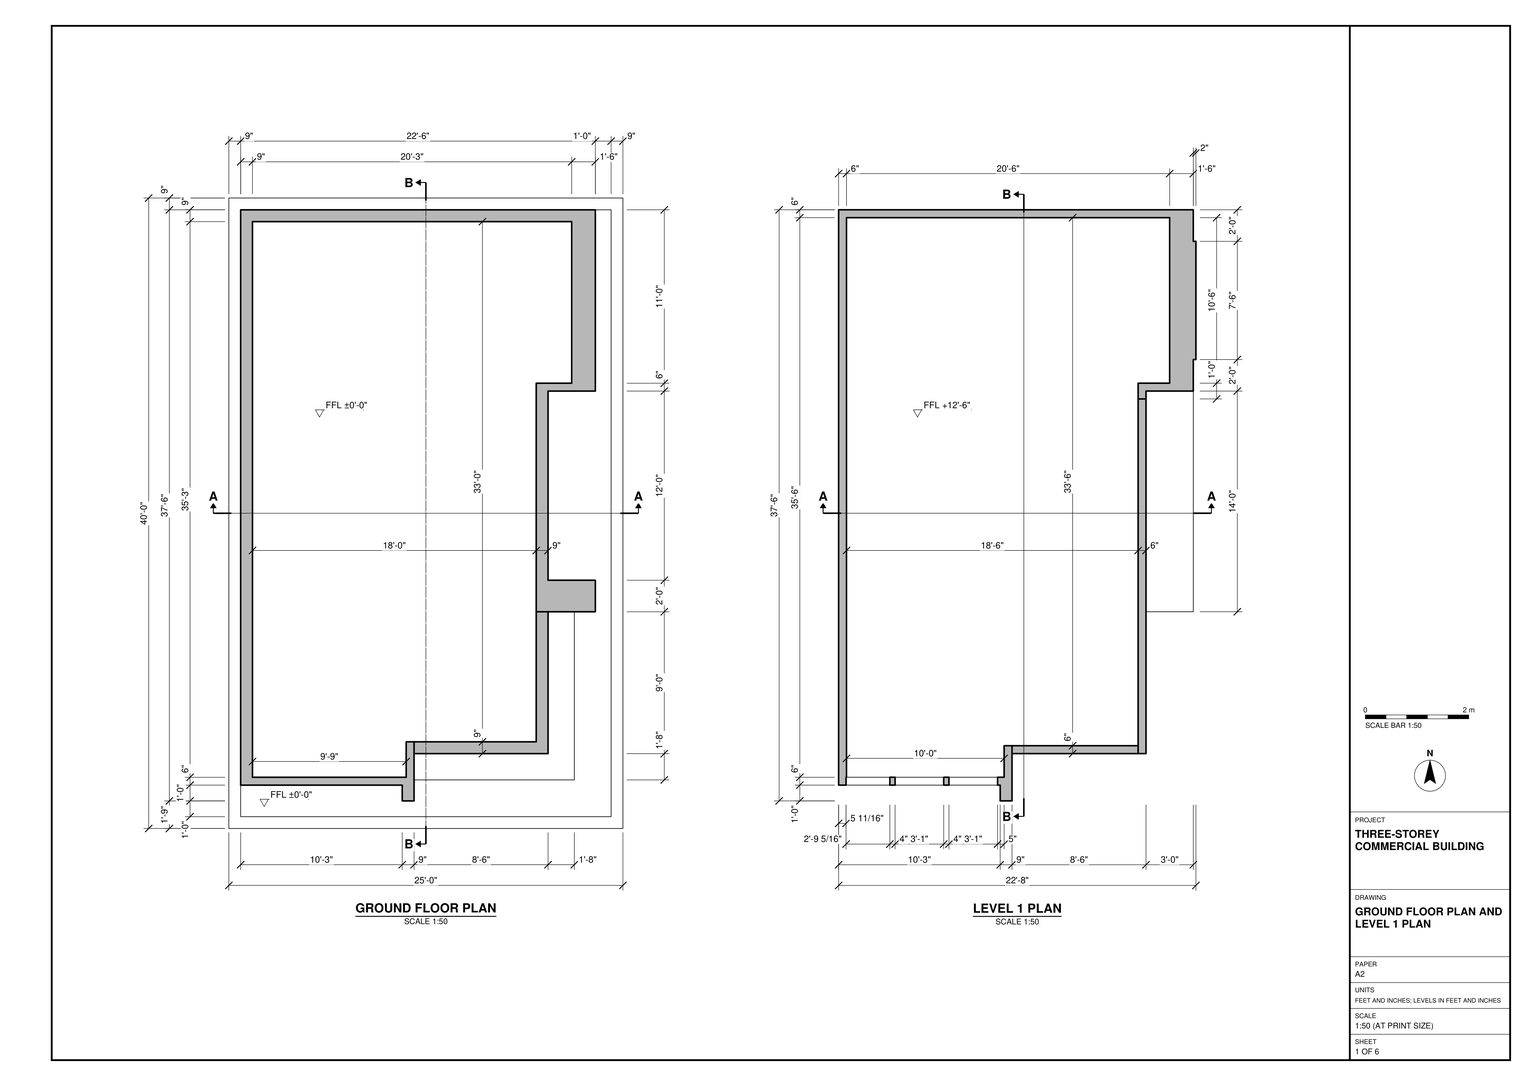
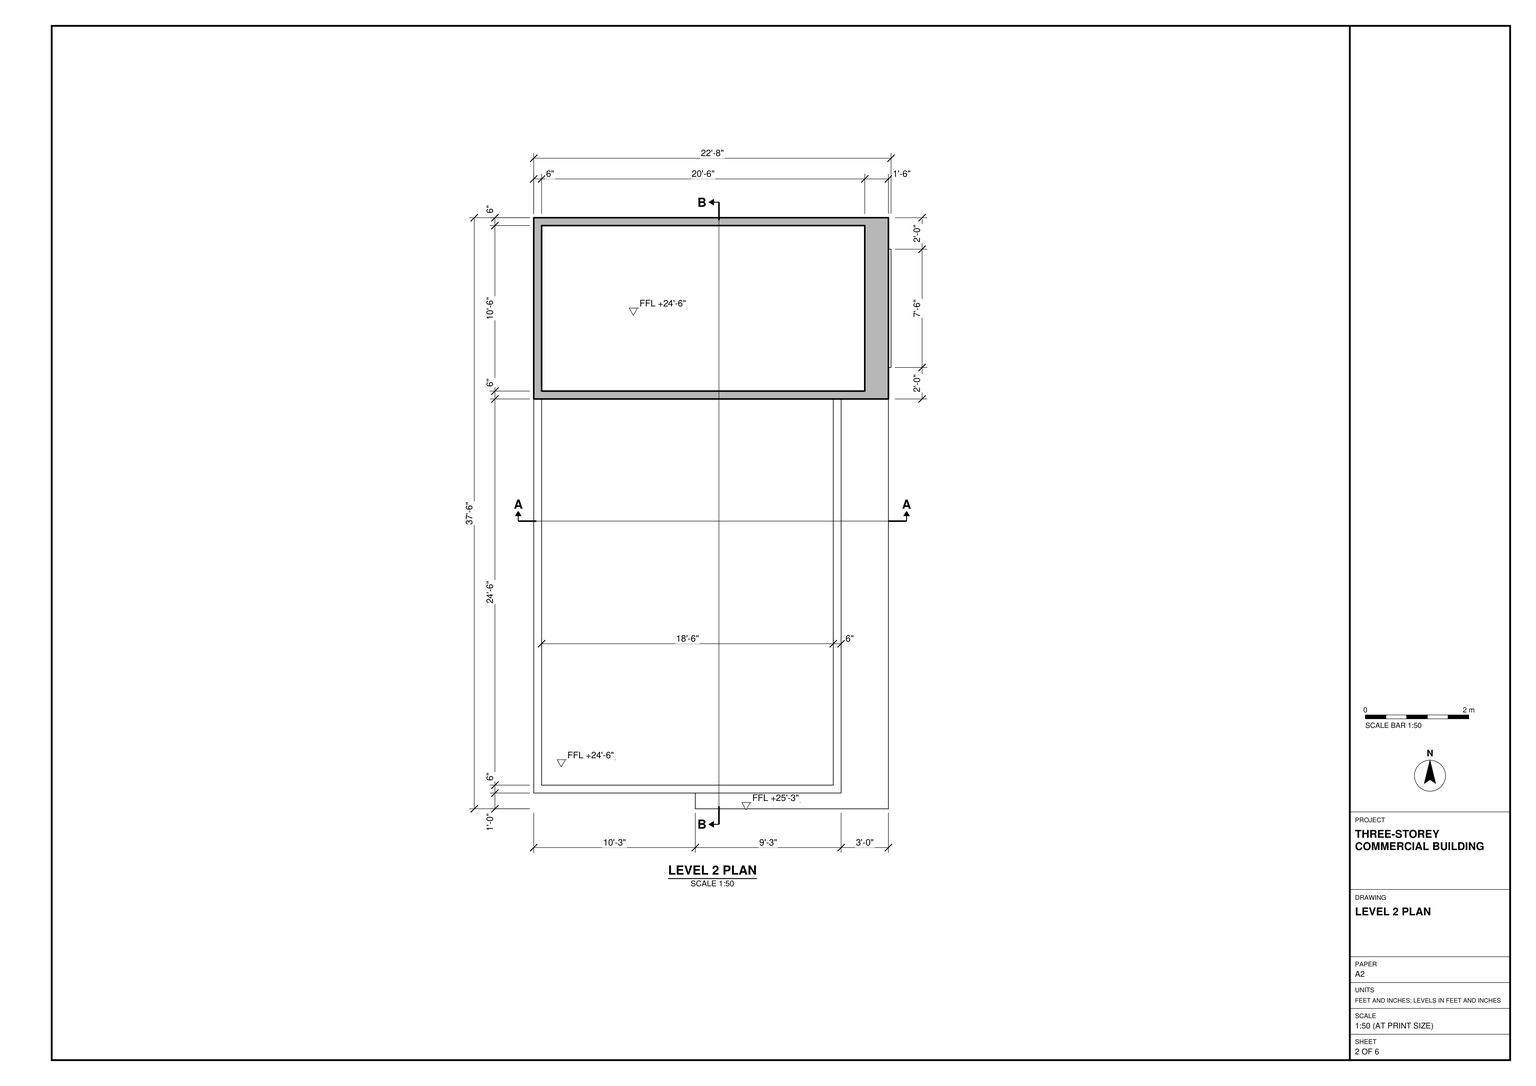
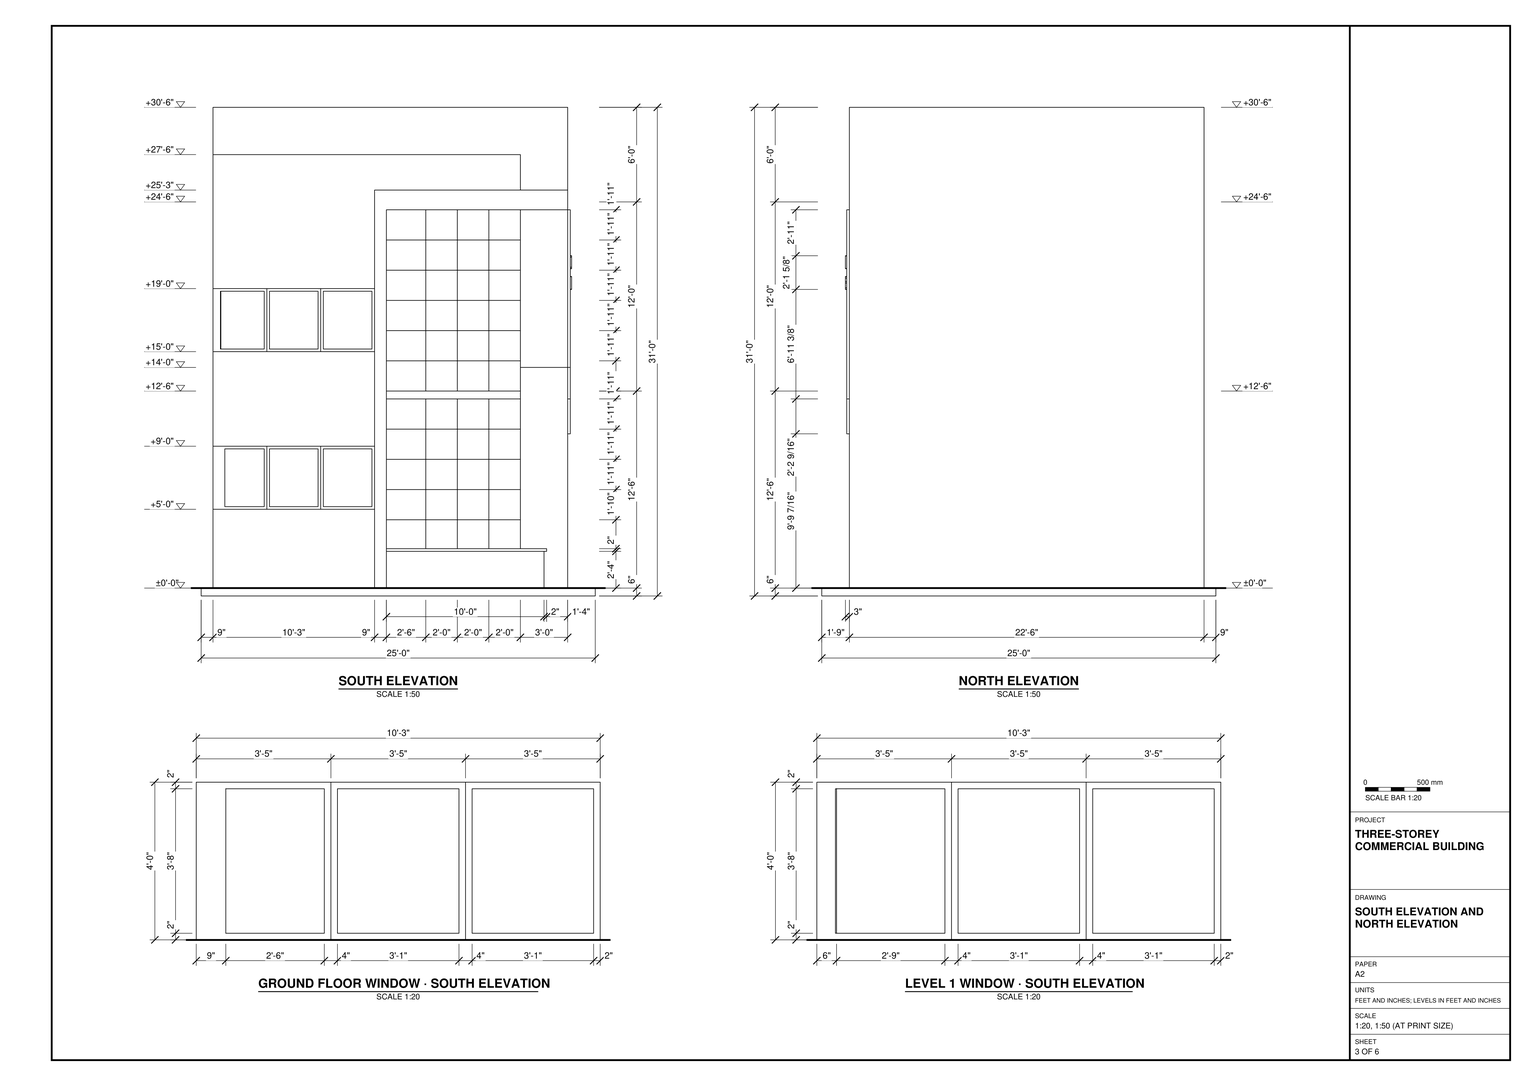
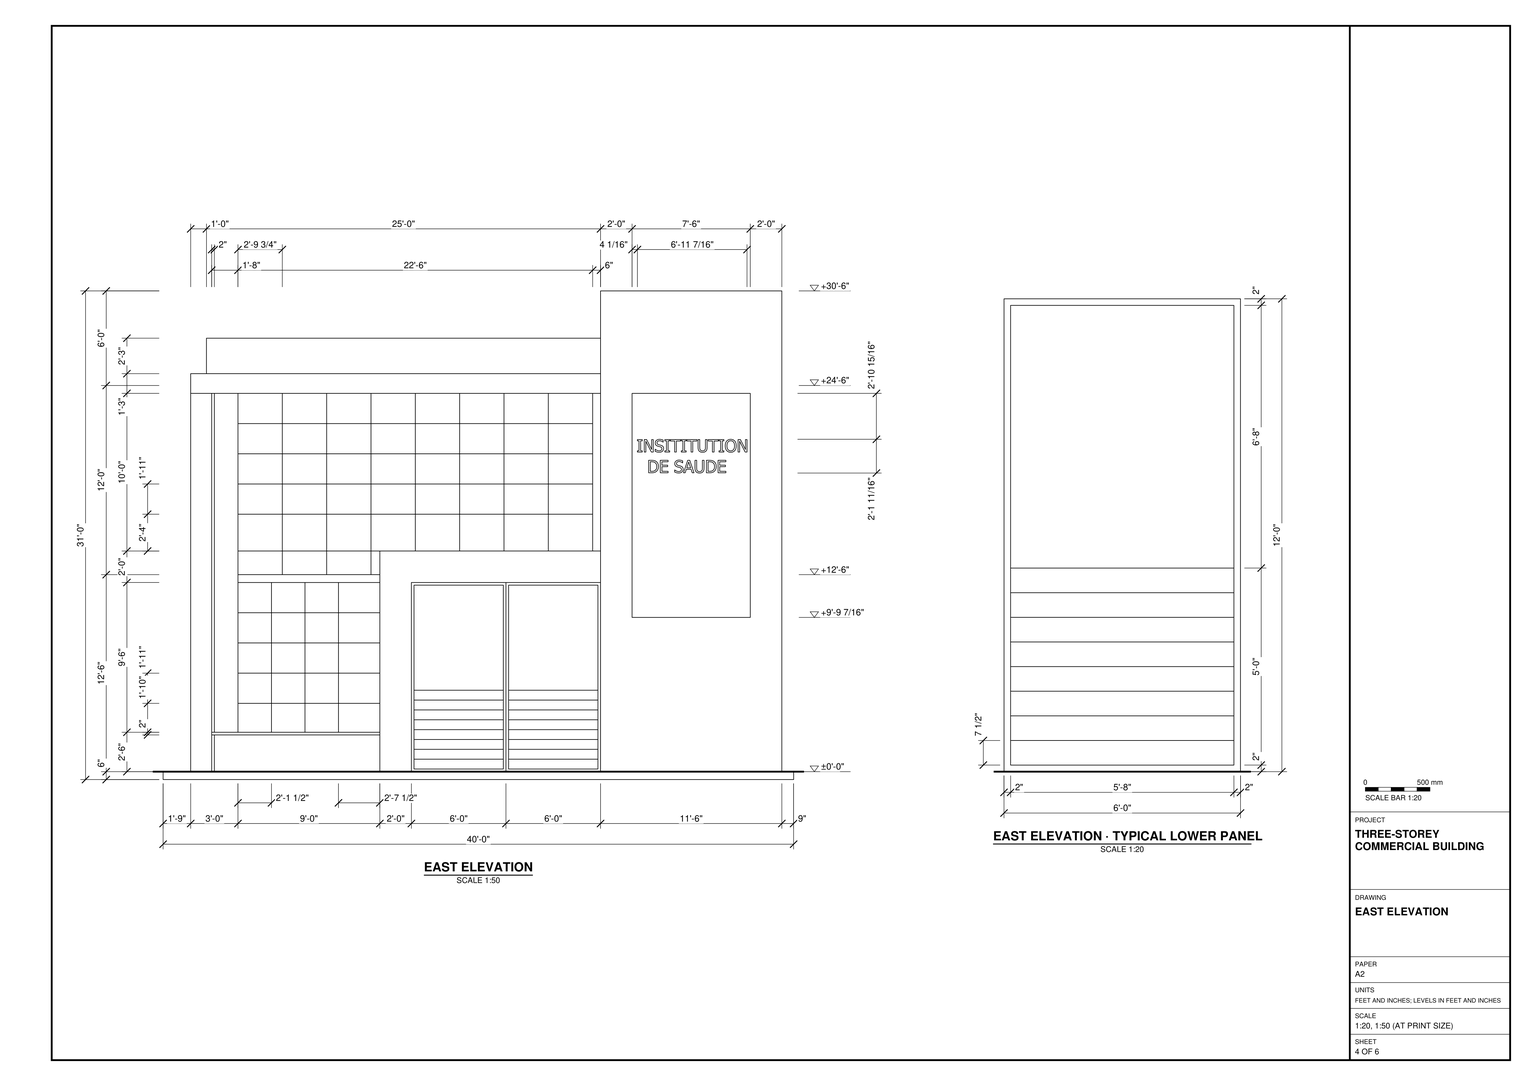
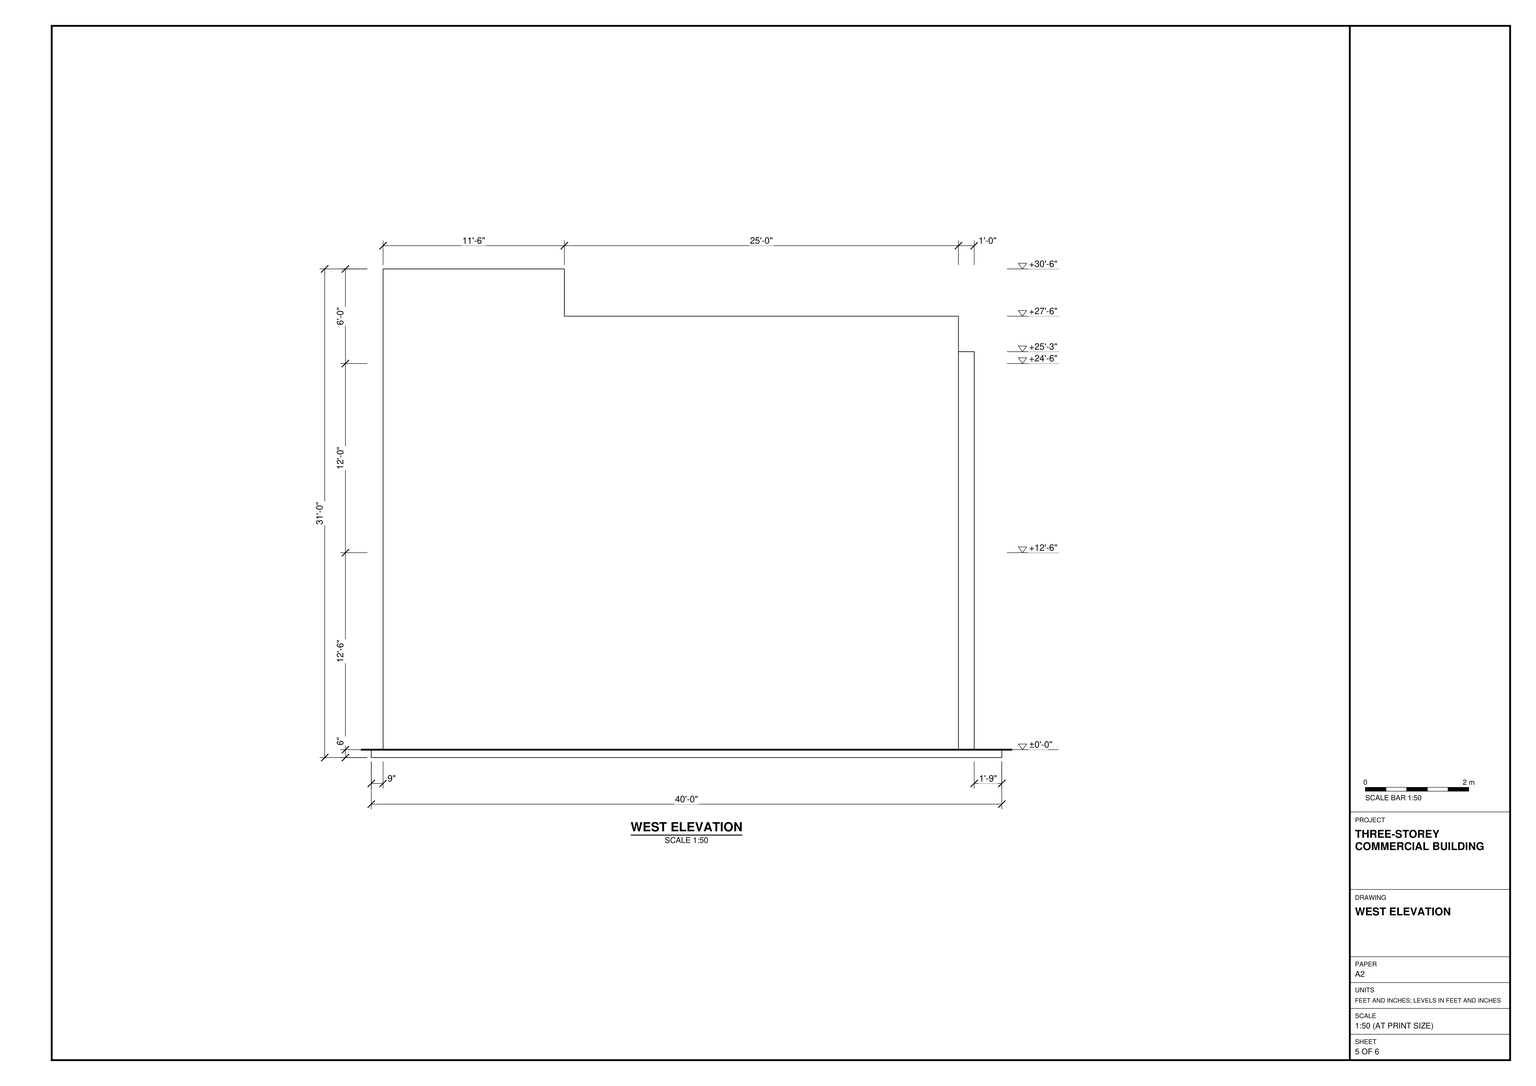
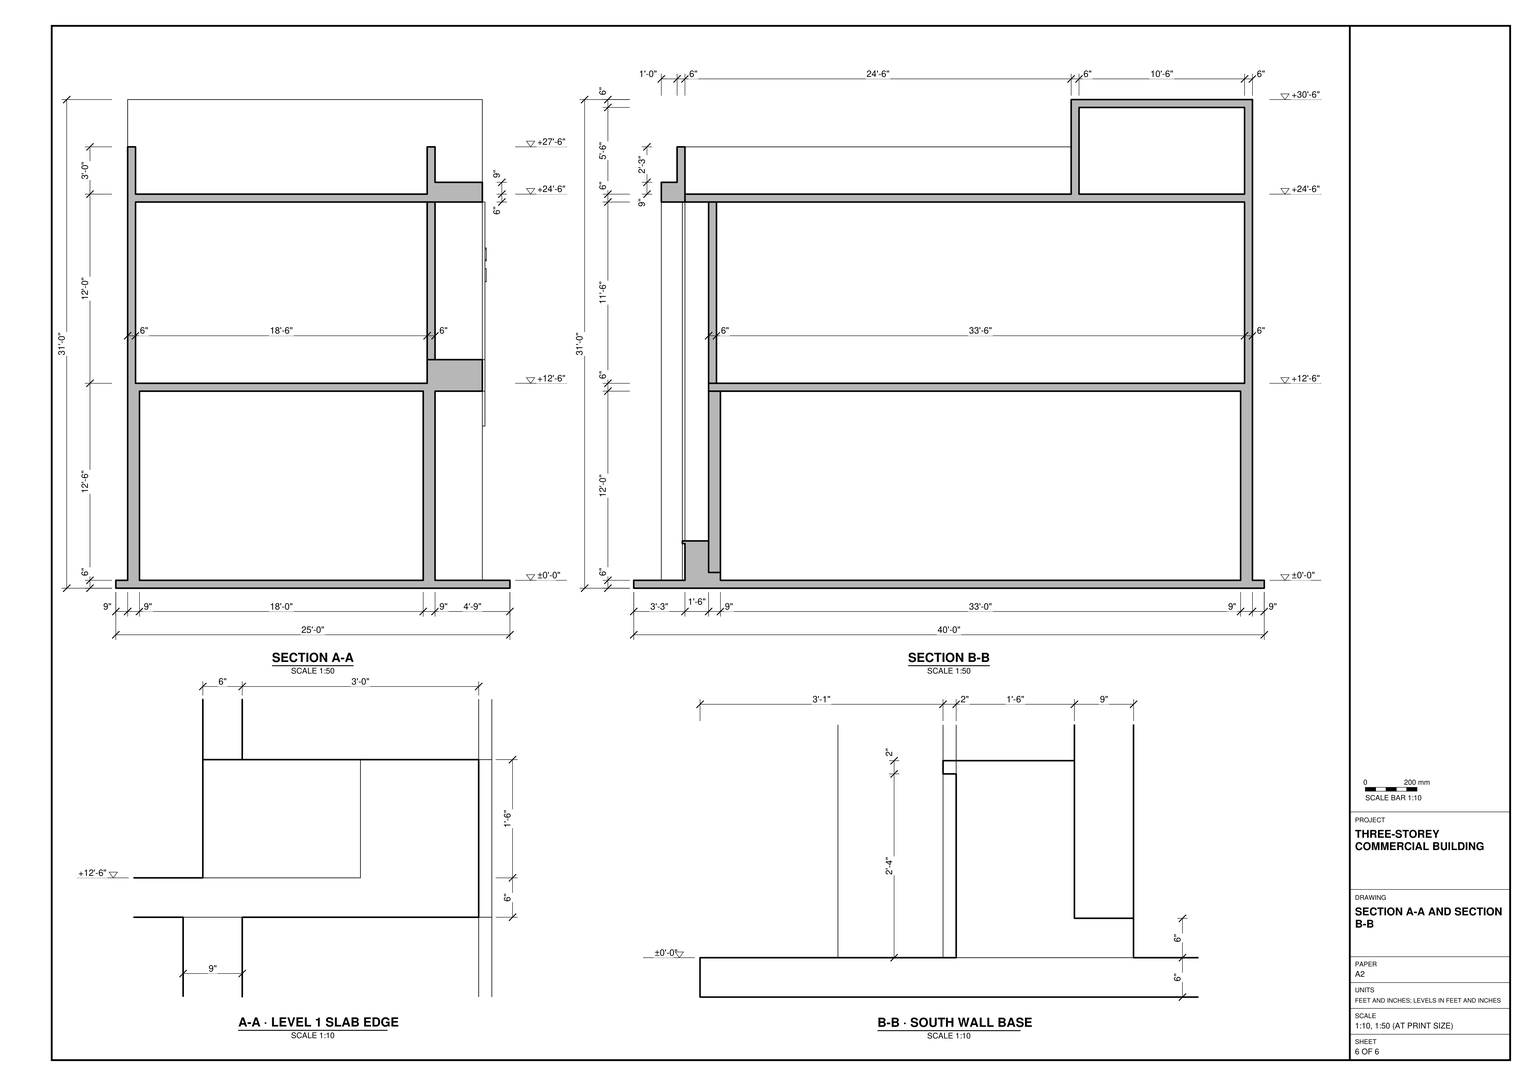
Work in feet and inches to model the three-storey commercial building in SketchUp from task_files/diagram_01.pdf. The overall dimensions, including the base slab, are 25'-0" wide along X, 40'-0" deep along Y and 31'-0" high along Z. Set the finished floor levels to ±0'-0", +12'-6" and +24'-6".

Set out the ground-floor walls on the projecting base slab. Follow the offsets in the east and south walls rather than using a rectangular footprint for every floor. Use the wall thicknesses shown in each plan, including the change in the west wall from 9" on the ground floor to 6" on level 1. Align the floor slabs and openings with these walls. At level 2, place the taller rectangular portion at the north end and the larger, lower roof area to its south.

Use the south elevation and window details to model the two bands of three framed panes. Beside them, model the tall gridded bay, its low base and its projecting surround. Keep the north elevation solid as drawn. Include stairs, built-in joinery and main furniture only where shown. Make the walls, slabs and roof separate groups or components, and group each furniture or joinery piece separately. Use components for repeated parts. Decor and loose items may be any suitable library components. Save one SketchUp model as output_files/three_storey_commercial_building_with_its_stepped_roof.skp.

# SketchUp Ruby script. Lengths in inches.
U = 1.inch
M = Sketchup.active_model
def pt(a) = Geom::Point3d.new(a.map { |v| v * U })
def face(e, loops, mat)
  f = e.add_face(loops[0].map { |a| pt(a) })
  loops[1..].each { |l| e.add_face(l.map { |a| pt(a) }).erase! }
  f.material = f.back_material = mat if mat
  f
end
# faces: each face lists its corners as indices into pts; further lists are holes
def faces(e, pts, list, mat = nil) = list.each { |f| face(e, (f[0].is_a?(Array) ? f : [f]).map { |l| l.map { |i| pts[i] } }, mat) }
# xy, xz, yz: faces in a plane at the given z, y or x. An outline is a flat list of corners, or four numbers for a rectangle; further outlines are holes
def ring(l) = l.size == 4 ? [[l[0], l[1]], [l[2], l[1]], [l[2], l[3]], [l[0], l[3]]] : l.each_slice(2).to_a
def flat(e, list, mat, &to3) = list.each { |f| face(e, (f[0].is_a?(Array) ? f : [f]).map { |l| ring(l).map { |u, v| to3.(u, v) } }, mat) }
def xy(e, z, list, mat = nil) = flat(e, list, mat) { |x, y| [x, y, z] }
def xz(e, y, list, mat = nil) = flat(e, list, mat) { |x, z| [x, y, z] }
def yz(e, x, list, mat = nil) = flat(e, list, mat) { |y, z| [x, y, z] }
def lines(e, pts, list) = list.each { |a, b| e.add_line(pt(pts[a]), pt(pts[b])) }
# prism: a flat outline (further loops are holes) pulled along v
def prism(e, loops, v, mat = nil)
  f = face(e, loops, mat); d = Geom::Vector3d.new(v.map { |x| x * U })
  f.pushpull(f.normal.samedirection?(d) ? d.length : -d.length)
end
def box(e, o, s, mat = nil) = prism(e, [[o, [o[0] + s[0], o[1], o[2]], [o[0] + s[0], o[1] + s[1], o[2]], [o[0], o[1] + s[1], o[2]]]], [0, 0, s[2]], mat)
def at(x, y, z, deg = 0) = Geom::Transformation.translation(pt([x, y, z])) * Geom::Transformation.rotation(ORIGIN, Z_AXIS, deg.degrees)
def axes(o, x, y, z) = Geom::Transformation.new([*x, 0, *y, 0, *z, 0, *pt(o).to_a, 1])
def part(name) = M.definitions.add(name)
# library, detail: a bought-in or finely detailed component or shape, given as its bounding box
def library(name, o, s) = part(name).tap { |d| box(d.entities, o, s) }
def detail(e, o, s) = box(e.add_group.entities, o, s)
def put(e, d, t, mat = nil) = e.add_instance(d, t).tap { |i| i.material = mat if mat }
def group(e, t, mat = nil) = e.add_group.tap { |g| g.transformation = t; g.material = mat if mat }.entities
root = M.entities
M.materials.add("D05_Goldenrod_Hue").color = [255, 191, 0]
M.materials.add("Glass_Basic_01").color = [64, 68, 73]
M.materials["Glass_Basic_01"].alpha = 0.25
M.materials.add("Plaster_04_1K").color = [183, 188, 179]
M.materials.add("Plywood_01_1K").color = [125, 96, 64]
M.materials.add("Wood_Veneer_15_1K").color = [103, 69, 45]
c1 = library("INSITITUTION   D",[0.59,0,0],[83.45,25.69,1])
xy(root,-6,[[0,0,300,480]])
xy(root,0,[[[0,0,300,480],[9,9,291,471]],[9,9,291,9,291,471,279,471,279,333,243,333,243,189,279,189,279,165,261,165,261,39,141,39,141,21,132,21,132,33,9,33],[18,39,135,39,135,66,234,66,234,339,261,339,261,462,18,462]])
xy(root,6,[[141,57,243,57,243,63,237,63,237,66,141,66],[237,63,243,63,243,165,234,165,234,66,237,66]])
xy(root,27.98,[[141,37,263,39],[261,39,263,165]])
xy(root,30,[[141,37,263,37,263,165,243,165,243,57,141,57]])
xy(root,62,[[18,33,48,39],[52,33,89,39],[93,33,130,39]])
xy(root,106,[[18,33,48,39],[52,33,89,39],[93,33,130,39]])
xy(root,117.42,[[279,357,281,447]],"Plywood_01_1K")
xy(root,144,[[18,39,18,462,261,462,261,339,234,339,234,66,135,66,135,39],[135,57,141,66],[141,57,141,66,234,66,234,165,243,165,243,57],[234,333,243,339],[243,333,261,339]])
xy(root,144,[[243,189,279,333]],"Plywood_01_1K")
xy(root,150,[[15,39,135,39,135,63,237,63,237,339,261,339,261,465,15,465],[141,57,237,63],[237,57,243,165]])
xy(root,168,[[237,165,243,327]])
xy(root,168,[[243,165,279,333]],"Plywood_01_1K")
xy(root,182,[[14.66,33,48,39],[52,33,89,39],[93,33,130,39]])
xy(root,226,[[14.66,33,48,39],[52,33,89,39],[93,33,130,39]])
xy(root,288,[[15,39,15,465,261,465,261,339,237,339,237,63,135,63,135,39],[141,57,237,63],[237,57,243,63],[237,63,243,327]])
xy(root,288,[[141,37,141,39,255,39,255,333,257,333,257,37]],"D05_Goldenrod_Hue")
xy(root,288,[[279,357,281,447]],"Plywood_01_1K")
xy(root,288,[[141,21,141,37,257,37,257,333,279,333,279,21],[141,39,141,57,243,57,243,333,255,333,255,39]],"Wood_Veneer_15_1K")
xy(root,294,[[15,339,261,465]])
xy(root,294,[[15,39,237,333]],"Wood_Veneer_15_1K")
xy(root,303,[[132,21,279,21,279,333,243,333,243,33,132,33]],"Wood_Veneer_15_1K")
xy(root,330,[[9,33,243,33,243,333,237,333,237,39,15,39,15,333,9,333]],"Plaster_04_1K")
xy(root,360,[[15,339,261,465]])
xy(root,366,[[9,333,279,471]],"Plaster_04_1K")
xz(root,0,[[0,-6,300,0]])
xz(root,21,[[132,0,141,0,141,288,279,288,279,303,132,303]],"Wood_Veneer_15_1K")
xz(root,33,[[[9,60,50,108],[18,62,48,106]],[[50,60,91,108],[52,62,89,106]],[[91,60,132,108],[93,62,130,106]],[9,108,132,180],[[9,180,50,228],[14.66,182,48,226]],
  [[50,180,91,228],[52,182,89,226]],[[91,180,132,228],[93,182,130,226]]])
xz(root,33,[[9,0,132,60],[9,228,132,228,132,303,243,303,243,330,9,330]],"Plaster_04_1K")
xz(root,37,[[141,27.98,263,30]])
xz(root,39,[[[18,0,18,62,48,62,48,106,18,106,18,144,135,144,135,0],[52,62,89,106],[93,62,130,106]],[[15,150,15,182,48,182,48,226,15,226,15,288,135,288,135,150],[52,182,89,226],[93,182,130,226]],[14.66,182,15,226],[141,288,237,294]])
xz(root,39,[[141,0,261,27.98],[15,294,237,330]],"Plaster_04_1K")
xz(root,57,[[141,6,171,29],[171,6,195,29],[195,6,219,29],[219,6,243,29],[141,29,171,30],
  [171,29,195,30],[195,29,219,30],[219,29,243,30],[141,30,171,52],[171,30,195,52],
  [195,30,219,52],[219,30,243,52],[141,52,171,75],[171,52,195,75],[195,52,219,75],
  [219,52,243,75],[141,75,171,98],[171,75,195,98],[195,75,219,98],[219,75,243,98],
  [141,98,171,121],[171,98,195,121],[195,98,219,121],[219,98,243,121],[141,121,171,144],
  [171,121,195,144],[195,121,219,144],[219,121,243,144],[141,150,171,173],[171,150,195,173],
  [195,150,219,173],[219,150,237,173],[237,150,243,173],[141,173,171,196],[171,173,195,196],
  [195,173,219,196],[219,173,237,196],[237,173,243,196],[141,196,171,219],[171,196,195,219],
  [195,196,219,219],[219,196,237,219],[237,196,243,219],[141,219,171,242],[171,219,195,242],
  [195,219,219,242],[219,219,237,242],[237,219,243,242],[141,242,171,265],[171,242,195,265],
  [195,242,219,265],[219,242,237,265],[237,242,243,265],[141,265,171,288],[171,265,195,288],
  [195,265,219,288],[219,265,237,288],[237,265,243,288]],"Glass_Basic_01")
xz(root,57,[[141,144,243,150]],"Plaster_04_1K")
xz(root,63,[[135,150,141,288]])
xz(root,63,[[141,150,237,288]],"Glass_Basic_01")
xz(root,66,[[135,0,141,144],[141,0,234,6]])
xz(root,66,[[141,6,234,144]],"Glass_Basic_01")
xz(root,165,[[234,6,243,144],[237,150,243,168]])
xz(root,165,[[261,0,279,0,279,168,243,168,243,30,263,30,263,27.98,261,27.98]],"Plywood_01_1K")
xz(root,189,[[243,0,279,144]],"Plywood_01_1K")
xz(root,327,[[237,168,243,288]])
xz(root,333,[[243,0,279,144],[243,168,279,288],[15,294,237,294,237,330,243,330,243,303,279,303,279,366,9,366,9,330,15,330]],"Plaster_04_1K")
xz(root,339,[[234,0,261,144],[237,150,261,288],[237,288,261,294],[15,294,237,360],[237,294,261,360]])
xz(root,357,[[279,117.42,281,144],[279,144,281,168],[279,168,281,288]],"Plywood_01_1K")
xz(root,447,[[279,117.42,281,144],[279,144,281,288]],"Plywood_01_1K")
xz(root,462,[[18,0,261,144]])
xz(root,465,[[15,150,261,288],[15,294,261,360]])
xz(root,471,[[9,0,279,366]])
xz(root,480,[[0,-6,300,0]])
yz(root,0,[[0,-6,480,0]])
yz(root,9,[[33,0,33,330,333,330,333,366,471,366,471,0]],"Plaster_04_1K")
yz(root,14.66,[[33,182,39,226]])
yz(root,15,[[39,150,465,288],[339,294,465,360]])
yz(root,15,[[39,294,333,330]],"Plaster_04_1K")
yz(root,18,[[39,0,462,144],[33,62,39,106]])
yz(root,48,[[33,62,39,106],[33,182,39,226]])
yz(root,52,[[33,62,39,106],[33,182,39,226]])
yz(root,89,[[33,62,39,106],[33,182,39,226]])
yz(root,93,[[33,62,39,106],[33,182,39,226]])
yz(root,130,[[33,62,39,106],[33,182,39,226]])
yz(root,132,[[21,0,33,303]],"Wood_Veneer_15_1K")
yz(root,135,[[39,0,66,144],[39,150,63,288]])
yz(root,141,[[57,6,66,144],[57,150,63,288]])
yz(root,141,[[37,0,39,27.98],[37,30,39,288]],"D05_Goldenrod_Hue")
yz(root,141,[[21,0,37,288],[39,30,57,288]],"Wood_Veneer_15_1K")
yz(root,234,[[66,0,66,6,165,6,165,144,333,144,333,0],[333,0,339,144]])
yz(root,234,[[66,6,165,144]],"Glass_Basic_01")
yz(root,237,[[165,150,165,168,327,168,327,288,339,288,339,150]])
yz(root,237,[[57,150,63,288],[63,150,63,288,327,288,327,168,165,168,165,150]],"Glass_Basic_01")
yz(root,237,[[39,294,333,330]],"Plaster_04_1K")
yz(root,243,[[57,29,63,30]])
yz(root,243,[[57,6,63,29],[63,6,82.5,29],[82.5,6,108,29],[108,6,133.5,29],[133.5,6,165,29],
  [63,29,82.5,30],[82.5,29,108,30],[108,29,133.5,30],[133.5,29,165,30],[57,30,82.5,52],
  [82.5,30,108,52],[108,30,133.5,52],[133.5,30,165,52],[57,52,82.5,75],[82.5,52,108,75],
  [108,52,133.5,75],[133.5,52,165,75],[57,75,82.5,98],[82.5,75,108,98],[108,75,133.5,98],
  [133.5,75,165,98],[57,98,82.5,121],[82.5,98,108,121],[108,98,133.5,121],[133.5,98,165,121],
  [57,121,82.5,144],[82.5,121,108,144],[108,121,133.5,144],[133.5,121,165,144],[57,150,90.75,168],
  [90.75,150,124.5,168],[124.5,150,158.25,168],[158.25,150,165,168],[57,168,90.75,196],[90.75,168,124.5,196],
  [124.5,168,158.25,196],[158.25,168,192,196],[192,168,225.75,196],[225.75,168,259.5,196],[259.5,168,293.25,196],
  [293.25,168,327,196],[57,196,90.75,219],[90.75,196,124.5,219],[124.5,196,158.25,219],[158.25,196,159,219],
  [159,196,192,219],[192,196,225.75,219],[225.75,196,259.5,219],[259.5,196,293.25,219],[293.25,196,327,219],
  [57,219,90.75,242],[90.75,219,124.5,242],[124.5,219,158.25,242],[158.25,219,159,242],[159,219,192,242],
  [192,219,225.75,242],[225.75,219,259.5,242],[259.5,219,293.25,242],[293.25,219,327,242],[57,242,90.75,265],
  [90.75,242,124.5,265],[124.5,242,158.25,265],[158.25,242,159,265],[159,242,192,265],[192,242,225.75,265],
  [225.75,242,259.5,265],[259.5,242,293.25,265],[293.25,242,327,265],[57,265,90.75,288],[90.75,265,124.5,288],
  [124.5,265,158.25,288],[158.25,265,159,288],[159,265,192,288],[192,265,225.75,288],[225.75,265,259.5,288],
  [259.5,265,293.25,288],[293.25,265,327,288]],"Glass_Basic_01")
yz(root,243,[[57,144,165,150],[327,168,333,288],[33,303,333,330]],"Plaster_04_1K")
yz(root,243,[[[189,0,261,144],[191,2,259,142]],[[261,0,333,144],[263,2,331,142]],[191,2,259,9.5],[263,2,331,9.5],[191,9.5,259,17],
  [263,9.5,331,17],[191,17,259,24.5],[263,17,331,24.5],[191,24.5,259,32],[263,24.5,331,32],
  [191,32,259,39.5],[263,32,331,39.5],[191,39.5,259,47],[263,39.5,331,47],[191,47,259,54.5],
  [263,47,331,54.5],[191,54.5,259,62],[263,54.5,331,62],[191,62,259,142],[263,62,331,142]],"Plywood_01_1K")
yz(root,261,[[339,0,462,144],[339,150,465,288],[339,294,465,360]])
yz(root,261,[[39,0,165,27.98]],"Plaster_04_1K")
yz(root,263,[[37,27.98,165,30]])
yz(root,279,[[[333,0,471,366],[357,117.42,447,288]]],"Plaster_04_1K")
yz(root,279,[[165,0,189,0,189,144,333,144,333,168,165,168]],"Plywood_01_1K")
yz(root,279,[[21,288,333,303]],"Wood_Veneer_15_1K")
yz(root,281,[[357,117.42,447,288]],"Plywood_01_1K")
yz(root,300,[[0,-6,480,0]])
p = [[18,462,144],[9,462,144],[18,39,144],[9,39,144],[135,39,288],[135,39,294],
  [243,333,294],[237,333,294],[132,42,0],[132,42,144],[132,42,294],[243,327,150],
  [243,165,150],[15,339,294],[15,333,294],[141,63,294],[141,63,288],[237,63,294],
  [237,63,288]]
lines(root,p,[[0,1],[2,3],[4,5],[6,7],[8,9],[9,10],[11,12],[13,14],[15,16],[17,18]])
put(root,c1,axes([281,360.47,227.35],[0,1,0],[0,0,1],[1,0,0]))
